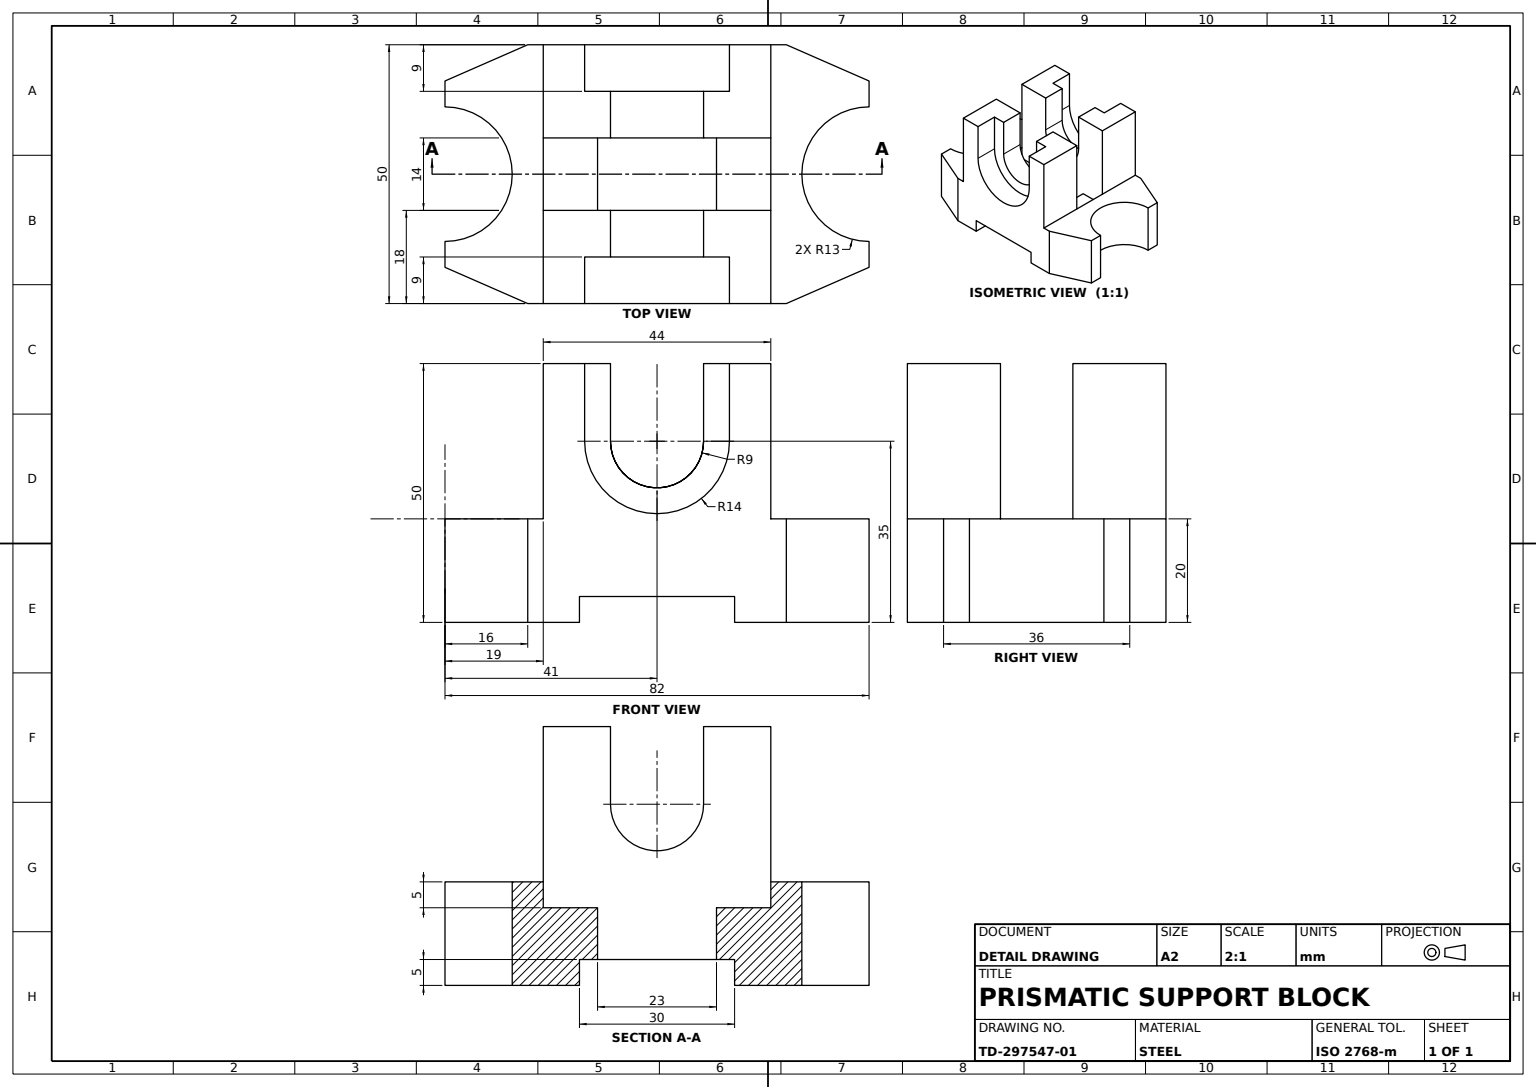
ISO-10303-21;
HEADER;
FILE_DESCRIPTION((''),'2;1');
FILE_NAME('','',(''),(''),'','','');
FILE_SCHEMA(('AUTOMOTIVE_DESIGN'));
ENDSEC;
DATA;
#1=APPLICATION_CONTEXT('');
#2=PRODUCT_CONTEXT('',#1,'mechanical');
#3=PRODUCT('','','',(#2));
#4=PRODUCT_DEFINITION_FORMATION('','',#3);
#5=PRODUCT_DEFINITION_CONTEXT('',#1,'design');
#6=PRODUCT_DEFINITION('','',#4,#5);
#7=PRODUCT_DEFINITION_SHAPE('','',#6);
#8=(LENGTH_UNIT()NAMED_UNIT(*)SI_UNIT(.MILLI.,.METRE.));
#9=(NAMED_UNIT(*)PLANE_ANGLE_UNIT()SI_UNIT($,.RADIAN.));
#10=(NAMED_UNIT(*)SI_UNIT($,.STERADIAN.)SOLID_ANGLE_UNIT());
#11=UNCERTAINTY_MEASURE_WITH_UNIT(LENGTH_MEASURE(1.E-05),#8,'distance_accuracy_value','');
#12=(GEOMETRIC_REPRESENTATION_CONTEXT(3)GLOBAL_UNCERTAINTY_ASSIGNED_CONTEXT((#11))GLOBAL_UNIT_ASSIGNED_CONTEXT((#8,#9,#10))REPRESENTATION_CONTEXT('',''));
#13=CARTESIAN_POINT('',(22.,20.,7.));
#14=VERTEX_POINT('',#13);
#15=CARTESIAN_POINT('',(22.,20.,25.));
#16=VERTEX_POINT('',#15);
#17=DIRECTION('',(0.,0.,1.));
#18=VECTOR('',#17,1000.);
#19=LINE('',#13,#18);
#20=EDGE_CURVE('',#14,#16,#19,.T.);
#21=ORIENTED_EDGE('',*,*,#20,.F.);
#22=CARTESIAN_POINT('',(22.,50.,7.));
#23=VERTEX_POINT('',#22);
#24=DIRECTION('',(0.,1.,0.));
#25=VECTOR('',#24,1000.);
#26=LINE('',#22,#25);
#27=EDGE_CURVE('',#14,#23,#26,.T.);
#28=ORIENTED_EDGE('',*,*,#27,.T.);
#29=CARTESIAN_POINT('',(22.,50.,25.));
#30=VERTEX_POINT('',#29);
#31=LINE('',#22,#18);
#32=EDGE_CURVE('',#23,#30,#31,.T.);
#33=ORIENTED_EDGE('',*,*,#32,.T.);
#34=LINE('',#29,#25);
#35=EDGE_CURVE('',#16,#30,#34,.T.);
#36=ORIENTED_EDGE('',*,*,#35,.F.);
#37=EDGE_LOOP('',(#21,#28,#33,#36));
#38=FACE_OUTER_BOUND('',#37,.T.);
#39=DIRECTION('',(1.,0.,0.));
#40=AXIS2_PLACEMENT_3D('',#22,#39,#24);
#41=PLANE('',#40);
#42=ADVANCED_FACE('',(#38),#41,.T.);
#43=CARTESIAN_POINT('',(14.,35.,-16.));
#44=VERTEX_POINT('',#43);
#45=CARTESIAN_POINT('',(14.,50.,-16.));
#46=VERTEX_POINT('',#45);
#47=LINE('',#45,#25);
#48=EDGE_CURVE('',#44,#46,#47,.T.);
#49=ORIENTED_EDGE('',*,*,#48,.T.);
#50=CARTESIAN_POINT('',(14.,50.,-25.));
#51=VERTEX_POINT('',#50);
#52=DIRECTION('',(0.,0.,-1.));
#53=VECTOR('',#52,1000.);
#54=LINE('',#45,#53);
#55=EDGE_CURVE('',#46,#51,#54,.T.);
#56=ORIENTED_EDGE('',*,*,#55,.T.);
#57=CARTESIAN_POINT('',(14.,35.,-25.));
#58=VERTEX_POINT('',#57);
#59=LINE('',#50,#25);
#60=EDGE_CURVE('',#58,#51,#59,.T.);
#61=ORIENTED_EDGE('',*,*,#60,.F.);
#62=LINE('',#43,#53);
#63=EDGE_CURVE('',#44,#58,#62,.T.);
#64=ORIENTED_EDGE('',*,*,#63,.F.);
#65=EDGE_LOOP('',(#49,#56,#61,#64));
#66=FACE_OUTER_BOUND('',#65,.T.);
#67=DIRECTION('',(-1.,0.,0.));
#68=DIRECTION('',(0.,-1.,0.));
#69=AXIS2_PLACEMENT_3D('',#45,#67,#68);
#70=PLANE('',#69);
#71=ADVANCED_FACE('',(#66),#70,.T.);
#72=CARTESIAN_POINT('',(15.,0.,25.));
#73=VERTEX_POINT('',#72);
#74=CARTESIAN_POINT('',(15.,5.,25.));
#75=VERTEX_POINT('',#74);
#76=CARTESIAN_POINT('',(15.,-5.,25.));
#77=LINE('',#76,#25);
#78=EDGE_CURVE('',#73,#75,#77,.T.);
#79=ORIENTED_EDGE('',*,*,#78,.T.);
#80=CARTESIAN_POINT('',(15.,5.,-25.));
#81=VERTEX_POINT('',#80);
#82=LINE('',#80,#18);
#83=EDGE_CURVE('',#81,#75,#82,.T.);
#84=ORIENTED_EDGE('',*,*,#83,.F.);
#85=CARTESIAN_POINT('',(15.,0.,-25.));
#86=VERTEX_POINT('',#85);
#87=CARTESIAN_POINT('',(15.,-5.,-25.));
#88=LINE('',#87,#25);
#89=EDGE_CURVE('',#86,#81,#88,.T.);
#90=ORIENTED_EDGE('',*,*,#89,.F.);
#91=CARTESIAN_POINT('',(15.,0.,0.));
#92=LINE('',#91,#18);
#93=EDGE_CURVE('',#86,#73,#92,.T.);
#94=ORIENTED_EDGE('',*,*,#93,.T.);
#95=EDGE_LOOP('',(#79,#84,#90,#94));
#96=FACE_OUTER_BOUND('',#95,.T.);
#97=AXIS2_PLACEMENT_3D('',#87,#39,#24);
#98=PLANE('',#97);
#99=ADVANCED_FACE('',(#96),#98,.F.);
#100=CARTESIAN_POINT('',(-22.,50.,-25.));
#101=VERTEX_POINT('',#100);
#102=CARTESIAN_POINT('',(-22.,20.,-25.));
#103=VERTEX_POINT('',#102);
#104=VECTOR('',#68,1000.);
#105=LINE('',#102,#104);
#106=EDGE_CURVE('',#101,#103,#105,.T.);
#107=ORIENTED_EDGE('',*,*,#106,.T.);
#108=CARTESIAN_POINT('',(-22.,20.,-7.));
#109=VERTEX_POINT('',#108);
#110=LINE('',#108,#53);
#111=EDGE_CURVE('',#109,#103,#110,.T.);
#112=ORIENTED_EDGE('',*,*,#111,.F.);
#113=CARTESIAN_POINT('',(-22.,50.,-7.));
#114=VERTEX_POINT('',#113);
#115=LINE('',#108,#104);
#116=EDGE_CURVE('',#114,#109,#115,.T.);
#117=ORIENTED_EDGE('',*,*,#116,.F.);
#118=LINE('',#113,#53);
#119=EDGE_CURVE('',#114,#101,#118,.T.);
#120=ORIENTED_EDGE('',*,*,#119,.T.);
#121=EDGE_LOOP('',(#107,#112,#117,#120));
#122=FACE_OUTER_BOUND('',#121,.T.);
#123=AXIS2_PLACEMENT_3D('',#108,#39,#52);
#124=PLANE('',#123);
#125=ADVANCED_FACE('',(#122),#124,.F.);
#126=CARTESIAN_POINT('',(-22.,15.,7.));
#127=VERTEX_POINT('',#126);
#128=CARTESIAN_POINT('',(-22.,20.,7.));
#129=VERTEX_POINT('',#128);
#130=LINE('',#126,#25);
#131=EDGE_CURVE('',#127,#129,#130,.T.);
#132=ORIENTED_EDGE('',*,*,#131,.F.);
#133=CARTESIAN_POINT('',(-22.,15.,-7.));
#134=VERTEX_POINT('',#133);
#135=LINE('',#133,#18);
#136=EDGE_CURVE('',#134,#127,#135,.T.);
#137=ORIENTED_EDGE('',*,*,#136,.F.);
#138=LINE('',#133,#25);
#139=EDGE_CURVE('',#134,#109,#138,.T.);
#140=ORIENTED_EDGE('',*,*,#139,.T.);
#141=LINE('',#108,#18);
#142=EDGE_CURVE('',#109,#129,#141,.T.);
#143=ORIENTED_EDGE('',*,*,#142,.T.);
#144=EDGE_LOOP('',(#132,#137,#140,#143));
#145=FACE_OUTER_BOUND('',#144,.T.);
#146=AXIS2_PLACEMENT_3D('',#133,#67,#17);
#147=PLANE('',#146);
#148=ADVANCED_FACE('',(#145),#147,.F.);
#149=CARTESIAN_POINT('',(-25.,0.,25.));
#150=VERTEX_POINT('',#149);
#151=CARTESIAN_POINT('',(-15.,0.,25.));
#152=VERTEX_POINT('',#151);
#153=CARTESIAN_POINT('',(25.,0.,25.));
#154=VECTOR('',#39,1000.);
#155=LINE('',#153,#154);
#156=EDGE_CURVE('',#150,#152,#155,.T.);
#157=ORIENTED_EDGE('',*,*,#156,.F.);
#158=CARTESIAN_POINT('',(-41.,0.,18.));
#159=VERTEX_POINT('',#158);
#160=DIRECTION('',(0.916157335,0.,0.400818834));
#161=VECTOR('',#160,1000.);
#162=LINE('',#158,#161);
#163=EDGE_CURVE('',#159,#150,#162,.T.);
#164=ORIENTED_EDGE('',*,*,#163,.F.);
#165=CARTESIAN_POINT('',(-41.,0.,13.));
#166=VERTEX_POINT('',#165);
#167=LINE('',#165,#18);
#168=EDGE_CURVE('',#166,#159,#167,.T.);
#169=ORIENTED_EDGE('',*,*,#168,.F.);
#170=CARTESIAN_POINT('',(-41.,0.,-13.));
#171=VERTEX_POINT('',#170);
#172=CARTESIAN_POINT('',(-41.,0.,0.));
#173=AXIS2_PLACEMENT_3D('',#172,#68,#52);
#174=CIRCLE('',#173,13.);
#175=EDGE_CURVE('',#171,#166,#174,.T.);
#176=ORIENTED_EDGE('',*,*,#175,.F.);
#177=CARTESIAN_POINT('',(-41.,0.,-18.));
#178=VERTEX_POINT('',#177);
#179=LINE('',#177,#18);
#180=EDGE_CURVE('',#178,#171,#179,.T.);
#181=ORIENTED_EDGE('',*,*,#180,.F.);
#182=CARTESIAN_POINT('',(-25.,0.,-25.));
#183=VERTEX_POINT('',#182);
#184=DIRECTION('',(-0.916157335,0.,0.400818834));
#185=VECTOR('',#184,1000.);
#186=LINE('',#182,#185);
#187=EDGE_CURVE('',#183,#178,#186,.T.);
#188=ORIENTED_EDGE('',*,*,#187,.F.);
#189=CARTESIAN_POINT('',(-15.,0.,-25.));
#190=VERTEX_POINT('',#189);
#191=VECTOR('',#67,1000.);
#192=LINE('',#182,#191);
#193=EDGE_CURVE('',#190,#183,#192,.T.);
#194=ORIENTED_EDGE('',*,*,#193,.F.);
#195=CARTESIAN_POINT('',(-15.,0.,0.));
#196=LINE('',#195,#53);
#197=EDGE_CURVE('',#152,#190,#196,.T.);
#198=ORIENTED_EDGE('',*,*,#197,.F.);
#199=EDGE_LOOP('',(#157,#164,#169,#176,#181,#188,#194,#198));
#200=FACE_OUTER_BOUND('',#199,.T.);
#201=PLANE('',#173);
#202=ADVANCED_FACE('',(#200),#201,.T.);
#203=VERTEX_POINT('',#153);
#204=EDGE_CURVE('',#73,#203,#155,.T.);
#205=ORIENTED_EDGE('',*,*,#204,.T.);
#206=CARTESIAN_POINT('',(25.,20.,25.));
#207=VERTEX_POINT('',#206);
#208=LINE('',#206,#104);
#209=EDGE_CURVE('',#207,#203,#208,.T.);
#210=ORIENTED_EDGE('',*,*,#209,.F.);
#211=LINE('',#206,#154);
#212=EDGE_CURVE('',#16,#207,#211,.T.);
#213=ORIENTED_EDGE('',*,*,#212,.F.);
#214=ORIENTED_EDGE('',*,*,#35,.T.);
#215=CARTESIAN_POINT('',(14.,50.,25.));
#216=VERTEX_POINT('',#215);
#217=CARTESIAN_POINT('',(9.,50.,25.));
#218=LINE('',#217,#191);
#219=EDGE_CURVE('',#30,#216,#218,.T.);
#220=ORIENTED_EDGE('',*,*,#219,.T.);
#221=CARTESIAN_POINT('',(14.,35.,25.));
#222=VERTEX_POINT('',#221);
#223=LINE('',#215,#25);
#224=EDGE_CURVE('',#222,#216,#223,.T.);
#225=ORIENTED_EDGE('',*,*,#224,.F.);
#226=CARTESIAN_POINT('',(-14.,35.,25.));
#227=VERTEX_POINT('',#226);
#228=CARTESIAN_POINT('',(0.,35.,25.));
#229=AXIS2_PLACEMENT_3D('',#228,#17,#39);
#230=CIRCLE('',#229,14.);
#231=EDGE_CURVE('',#227,#222,#230,.T.);
#232=ORIENTED_EDGE('',*,*,#231,.F.);
#233=CARTESIAN_POINT('',(-14.,50.,25.));
#234=VERTEX_POINT('',#233);
#235=LINE('',#226,#104);
#236=EDGE_CURVE('',#234,#227,#235,.T.);
#237=ORIENTED_EDGE('',*,*,#236,.F.);
#238=CARTESIAN_POINT('',(-22.,50.,25.));
#239=VERTEX_POINT('',#238);
#240=LINE('',#238,#191);
#241=EDGE_CURVE('',#234,#239,#240,.T.);
#242=ORIENTED_EDGE('',*,*,#241,.T.);
#243=CARTESIAN_POINT('',(-22.,20.,25.));
#244=VERTEX_POINT('',#243);
#245=LINE('',#243,#104);
#246=EDGE_CURVE('',#239,#244,#245,.T.);
#247=ORIENTED_EDGE('',*,*,#246,.T.);
#248=CARTESIAN_POINT('',(-25.,20.,25.));
#249=VERTEX_POINT('',#248);
#250=EDGE_CURVE('',#249,#244,#211,.T.);
#251=ORIENTED_EDGE('',*,*,#250,.F.);
#252=LINE('',#248,#104);
#253=EDGE_CURVE('',#249,#150,#252,.T.);
#254=ORIENTED_EDGE('',*,*,#253,.T.);
#255=ORIENTED_EDGE('',*,*,#156,.T.);
#256=CARTESIAN_POINT('',(-15.,5.,25.));
#257=VERTEX_POINT('',#256);
#258=CARTESIAN_POINT('',(-15.,-5.,25.));
#259=LINE('',#258,#104);
#260=EDGE_CURVE('',#257,#152,#259,.T.);
#261=ORIENTED_EDGE('',*,*,#260,.F.);
#262=LINE('',#256,#191);
#263=EDGE_CURVE('',#75,#257,#262,.T.);
#264=ORIENTED_EDGE('',*,*,#263,.F.);
#265=ORIENTED_EDGE('',*,*,#78,.F.);
#266=EDGE_LOOP('',(#205,#210,#213,#214,#220,#225,#232,#237,#242,#247,#251,#254,#255,#261,#264,#265));
#267=FACE_OUTER_BOUND('',#266,.T.);
#268=AXIS2_PLACEMENT_3D('',#206,#52,#67);
#269=PLANE('',#268);
#270=ADVANCED_FACE('',(#267),#269,.F.);
#271=CARTESIAN_POINT('',(-11.5,5.,7.));
#272=VERTEX_POINT('',#271);
#273=CARTESIAN_POINT('',(-11.5,15.,7.));
#274=VERTEX_POINT('',#273);
#275=CARTESIAN_POINT('',(-11.5,0.,7.));
#276=LINE('',#275,#25);
#277=EDGE_CURVE('',#272,#274,#276,.T.);
#278=ORIENTED_EDGE('',*,*,#277,.F.);
#279=CARTESIAN_POINT('',(-11.5,5.,-7.));
#280=VERTEX_POINT('',#279);
#281=CARTESIAN_POINT('',(-11.5,5.,-25.));
#282=LINE('',#281,#18);
#283=EDGE_CURVE('',#280,#272,#282,.T.);
#284=ORIENTED_EDGE('',*,*,#283,.F.);
#285=CARTESIAN_POINT('',(-11.5,15.,-7.));
#286=VERTEX_POINT('',#285);
#287=CARTESIAN_POINT('',(-11.5,0.,-7.));
#288=LINE('',#287,#25);
#289=EDGE_CURVE('',#280,#286,#288,.T.);
#290=ORIENTED_EDGE('',*,*,#289,.T.);
#291=LINE('',#273,#53);
#292=EDGE_CURVE('',#274,#286,#291,.T.);
#293=ORIENTED_EDGE('',*,*,#292,.F.);
#294=EDGE_LOOP('',(#278,#284,#290,#293));
#295=FACE_OUTER_BOUND('',#294,.T.);
#296=AXIS2_PLACEMENT_3D('',#275,#67,#17);
#297=PLANE('',#296);
#298=ADVANCED_FACE('',(#295),#297,.F.);
#299=CARTESIAN_POINT('',(9.,35.,-16.));
#300=VERTEX_POINT('',#299);
#301=CARTESIAN_POINT('',(9.,50.,-16.));
#302=VERTEX_POINT('',#301);
#303=LINE('',#299,#25);
#304=EDGE_CURVE('',#300,#302,#303,.T.);
#305=ORIENTED_EDGE('',*,*,#304,.F.);
#306=CARTESIAN_POINT('',(9.,35.,-7.));
#307=VERTEX_POINT('',#306);
#308=LINE('',#306,#53);
#309=EDGE_CURVE('',#307,#300,#308,.T.);
#310=ORIENTED_EDGE('',*,*,#309,.F.);
#311=CARTESIAN_POINT('',(9.,50.,-7.));
#312=VERTEX_POINT('',#311);
#313=LINE('',#306,#104);
#314=EDGE_CURVE('',#312,#307,#313,.T.);
#315=ORIENTED_EDGE('',*,*,#314,.F.);
#316=LINE('',#311,#53);
#317=EDGE_CURVE('',#312,#302,#316,.T.);
#318=ORIENTED_EDGE('',*,*,#317,.T.);
#319=EDGE_LOOP('',(#305,#310,#315,#318));
#320=FACE_OUTER_BOUND('',#319,.T.);
#321=AXIS2_PLACEMENT_3D('',#306,#39,#24);
#322=PLANE('',#321);
#323=ADVANCED_FACE('',(#320),#322,.F.);
#324=CARTESIAN_POINT('',(22.,15.,-7.));
#325=VERTEX_POINT('',#324);
#326=CARTESIAN_POINT('',(22.,20.,-7.));
#327=VERTEX_POINT('',#326);
#328=LINE('',#324,#25);
#329=EDGE_CURVE('',#325,#327,#328,.T.);
#330=ORIENTED_EDGE('',*,*,#329,.F.);
#331=CARTESIAN_POINT('',(22.,15.,7.));
#332=VERTEX_POINT('',#331);
#333=LINE('',#324,#53);
#334=EDGE_CURVE('',#332,#325,#333,.T.);
#335=ORIENTED_EDGE('',*,*,#334,.F.);
#336=LINE('',#331,#25);
#337=EDGE_CURVE('',#332,#14,#336,.T.);
#338=ORIENTED_EDGE('',*,*,#337,.T.);
#339=LINE('',#326,#53);
#340=EDGE_CURVE('',#14,#327,#339,.T.);
#341=ORIENTED_EDGE('',*,*,#340,.T.);
#342=EDGE_LOOP('',(#330,#335,#338,#341));
#343=FACE_OUTER_BOUND('',#342,.T.);
#344=AXIS2_PLACEMENT_3D('',#324,#39,#52);
#345=PLANE('',#344);
#346=ADVANCED_FACE('',(#343),#345,.F.);
#347=CARTESIAN_POINT('',(9.,50.,7.));
#348=VERTEX_POINT('',#347);
#349=CARTESIAN_POINT('',(9.,50.,16.));
#350=VERTEX_POINT('',#349);
#351=LINE('',#347,#18);
#352=EDGE_CURVE('',#348,#350,#351,.T.);
#353=ORIENTED_EDGE('',*,*,#352,.F.);
#354=CARTESIAN_POINT('',(9.,35.,7.));
#355=VERTEX_POINT('',#354);
#356=LINE('',#354,#104);
#357=EDGE_CURVE('',#348,#355,#356,.T.);
#358=ORIENTED_EDGE('',*,*,#357,.T.);
#359=CARTESIAN_POINT('',(9.,35.,16.));
#360=VERTEX_POINT('',#359);
#361=LINE('',#354,#18);
#362=EDGE_CURVE('',#355,#360,#361,.T.);
#363=ORIENTED_EDGE('',*,*,#362,.T.);
#364=LINE('',#359,#25);
#365=EDGE_CURVE('',#360,#350,#364,.T.);
#366=ORIENTED_EDGE('',*,*,#365,.T.);
#367=EDGE_LOOP('',(#353,#358,#363,#366));
#368=FACE_OUTER_BOUND('',#367,.T.);
#369=AXIS2_PLACEMENT_3D('',#354,#67,#68);
#370=PLANE('',#369);
#371=ADVANCED_FACE('',(#368),#370,.T.);
#372=CARTESIAN_POINT('',(-9.,50.,7.));
#373=VERTEX_POINT('',#372);
#374=CARTESIAN_POINT('',(-9.,50.,16.));
#375=VERTEX_POINT('',#374);
#376=LINE('',#372,#18);
#377=EDGE_CURVE('',#373,#375,#376,.T.);
#378=ORIENTED_EDGE('',*,*,#377,.T.);
#379=CARTESIAN_POINT('',(-9.,35.,16.));
#380=VERTEX_POINT('',#379);
#381=LINE('',#374,#104);
#382=EDGE_CURVE('',#375,#380,#381,.T.);
#383=ORIENTED_EDGE('',*,*,#382,.T.);
#384=CARTESIAN_POINT('',(-9.,35.,7.));
#385=VERTEX_POINT('',#384);
#386=LINE('',#384,#18);
#387=EDGE_CURVE('',#385,#380,#386,.T.);
#388=ORIENTED_EDGE('',*,*,#387,.F.);
#389=LINE('',#372,#25);
#390=EDGE_CURVE('',#385,#373,#389,.T.);
#391=ORIENTED_EDGE('',*,*,#390,.T.);
#392=EDGE_LOOP('',(#378,#383,#388,#391));
#393=FACE_OUTER_BOUND('',#392,.T.);
#394=AXIS2_PLACEMENT_3D('',#372,#39,#24);
#395=PLANE('',#394);
#396=ADVANCED_FACE('',(#393),#395,.T.);
#397=CARTESIAN_POINT('',(14.,50.,16.));
#398=VERTEX_POINT('',#397);
#399=CARTESIAN_POINT('',(-14.,50.,16.));
#400=LINE('',#399,#191);
#401=EDGE_CURVE('',#398,#350,#400,.T.);
#402=ORIENTED_EDGE('',*,*,#401,.F.);
#403=LINE('',#397,#18);
#404=EDGE_CURVE('',#398,#216,#403,.T.);
#405=ORIENTED_EDGE('',*,*,#404,.T.);
#406=ORIENTED_EDGE('',*,*,#219,.F.);
#407=ORIENTED_EDGE('',*,*,#32,.F.);
#408=LINE('',#347,#191);
#409=EDGE_CURVE('',#23,#348,#408,.T.);
#410=ORIENTED_EDGE('',*,*,#409,.T.);
#411=ORIENTED_EDGE('',*,*,#352,.T.);
#412=EDGE_LOOP('',(#402,#405,#406,#407,#410,#411));
#413=FACE_OUTER_BOUND('',#412,.T.);
#414=AXIS2_PLACEMENT_3D('',#347,#24,#17);
#415=PLANE('',#414);
#416=ADVANCED_FACE('',(#413),#415,.T.);
#417=CARTESIAN_POINT('',(41.,0.,13.));
#418=VERTEX_POINT('',#417);
#419=CARTESIAN_POINT('',(41.,0.,-13.));
#420=VERTEX_POINT('',#419);
#421=CARTESIAN_POINT('',(41.,0.,0.));
#422=AXIS2_PLACEMENT_3D('',#421,#68,#17);
#423=CIRCLE('',#422,13.);
#424=EDGE_CURVE('',#418,#420,#423,.T.);
#425=ORIENTED_EDGE('',*,*,#424,.T.);
#426=CARTESIAN_POINT('',(41.,20.,-13.));
#427=VERTEX_POINT('',#426);
#428=LINE('',#426,#104);
#429=EDGE_CURVE('',#427,#420,#428,.T.);
#430=ORIENTED_EDGE('',*,*,#429,.F.);
#431=CARTESIAN_POINT('',(41.,20.,13.));
#432=VERTEX_POINT('',#431);
#433=CARTESIAN_POINT('',(41.,20.,0.));
#434=AXIS2_PLACEMENT_3D('',#433,#68,#17);
#435=CIRCLE('',#434,13.);
#436=EDGE_CURVE('',#432,#427,#435,.T.);
#437=ORIENTED_EDGE('',*,*,#436,.F.);
#438=LINE('',#431,#104);
#439=EDGE_CURVE('',#432,#418,#438,.T.);
#440=ORIENTED_EDGE('',*,*,#439,.T.);
#441=EDGE_LOOP('',(#425,#430,#437,#440));
#442=FACE_OUTER_BOUND('',#441,.T.);
#443=AXIS2_PLACEMENT_3D('',#433,#68,#52);
#444=CYLINDRICAL_SURFACE('',#443,13.);
#445=ADVANCED_FACE('',(#442),#444,.F.);
#446=CARTESIAN_POINT('',(22.,20.,-25.));
#447=VERTEX_POINT('',#446);
#448=CARTESIAN_POINT('',(22.,50.,-25.));
#449=VERTEX_POINT('',#448);
#450=LINE('',#448,#25);
#451=EDGE_CURVE('',#447,#449,#450,.T.);
#452=ORIENTED_EDGE('',*,*,#451,.T.);
#453=CARTESIAN_POINT('',(22.,50.,-7.));
#454=VERTEX_POINT('',#453);
#455=LINE('',#453,#53);
#456=EDGE_CURVE('',#454,#449,#455,.T.);
#457=ORIENTED_EDGE('',*,*,#456,.F.);
#458=LINE('',#453,#25);
#459=EDGE_CURVE('',#327,#454,#458,.T.);
#460=ORIENTED_EDGE('',*,*,#459,.F.);
#461=EDGE_CURVE('',#327,#447,#339,.T.);
#462=ORIENTED_EDGE('',*,*,#461,.T.);
#463=EDGE_LOOP('',(#452,#457,#460,#462));
#464=FACE_OUTER_BOUND('',#463,.T.);
#465=AXIS2_PLACEMENT_3D('',#453,#67,#68);
#466=PLANE('',#465);
#467=ADVANCED_FACE('',(#464),#466,.F.);
#468=CARTESIAN_POINT('',(11.5,15.,-7.));
#469=VERTEX_POINT('',#468);
#470=CARTESIAN_POINT('',(11.5,15.,7.));
#471=VERTEX_POINT('',#470);
#472=LINE('',#470,#18);
#473=EDGE_CURVE('',#469,#471,#472,.T.);
#474=ORIENTED_EDGE('',*,*,#473,.F.);
#475=CARTESIAN_POINT('',(11.5,5.,-7.));
#476=VERTEX_POINT('',#475);
#477=CARTESIAN_POINT('',(11.5,0.,-7.));
#478=LINE('',#477,#25);
#479=EDGE_CURVE('',#476,#469,#478,.T.);
#480=ORIENTED_EDGE('',*,*,#479,.F.);
#481=CARTESIAN_POINT('',(11.5,5.,7.));
#482=VERTEX_POINT('',#481);
#483=CARTESIAN_POINT('',(11.5,5.,-25.));
#484=LINE('',#483,#53);
#485=EDGE_CURVE('',#482,#476,#484,.T.);
#486=ORIENTED_EDGE('',*,*,#485,.F.);
#487=CARTESIAN_POINT('',(11.5,0.,7.));
#488=LINE('',#487,#25);
#489=EDGE_CURVE('',#482,#471,#488,.T.);
#490=ORIENTED_EDGE('',*,*,#489,.T.);
#491=EDGE_LOOP('',(#474,#480,#486,#490));
#492=FACE_OUTER_BOUND('',#491,.T.);
#493=AXIS2_PLACEMENT_3D('',#487,#39,#52);
#494=PLANE('',#493);
#495=ADVANCED_FACE('',(#492),#494,.F.);
#496=ORIENTED_EDGE('',*,*,#163,.T.);
#497=ORIENTED_EDGE('',*,*,#253,.F.);
#498=CARTESIAN_POINT('',(-41.,20.,18.));
#499=VERTEX_POINT('',#498);
#500=LINE('',#498,#161);
#501=EDGE_CURVE('',#499,#249,#500,.T.);
#502=ORIENTED_EDGE('',*,*,#501,.F.);
#503=LINE('',#498,#104);
#504=EDGE_CURVE('',#499,#159,#503,.T.);
#505=ORIENTED_EDGE('',*,*,#504,.T.);
#506=EDGE_LOOP('',(#496,#497,#502,#505));
#507=FACE_OUTER_BOUND('',#506,.T.);
#508=DIRECTION('',(0.400818834,0.,-0.916157335));
#509=DIRECTION('',(-0.916157335,0.,-0.400818834));
#510=AXIS2_PLACEMENT_3D('',#498,#508,#509);
#511=PLANE('',#510);
#512=ADVANCED_FACE('',(#507),#511,.F.);
#513=CARTESIAN_POINT('',(-14.,35.,16.));
#514=VERTEX_POINT('',#513);
#515=LINE('',#513,#18);
#516=EDGE_CURVE('',#514,#227,#515,.T.);
#517=ORIENTED_EDGE('',*,*,#516,.T.);
#518=ORIENTED_EDGE('',*,*,#231,.T.);
#519=CARTESIAN_POINT('',(14.,35.,16.));
#520=VERTEX_POINT('',#519);
#521=LINE('',#519,#18);
#522=EDGE_CURVE('',#520,#222,#521,.T.);
#523=ORIENTED_EDGE('',*,*,#522,.F.);
#524=CARTESIAN_POINT('',(0.,35.,16.));
#525=AXIS2_PLACEMENT_3D('',#524,#17,#39);
#526=CIRCLE('',#525,14.);
#527=EDGE_CURVE('',#514,#520,#526,.T.);
#528=ORIENTED_EDGE('',*,*,#527,.F.);
#529=EDGE_LOOP('',(#517,#518,#523,#528));
#530=FACE_OUTER_BOUND('',#529,.T.);
#531=CYLINDRICAL_SURFACE('',#525,14.);
#532=ADVANCED_FACE('',(#530),#531,.F.);
#533=CARTESIAN_POINT('',(-15.,5.,-25.));
#534=VERTEX_POINT('',#533);
#535=LINE('',#533,#18);
#536=EDGE_CURVE('',#534,#257,#535,.T.);
#537=ORIENTED_EDGE('',*,*,#536,.F.);
#538=LINE('',#533,#191);
#539=EDGE_CURVE('',#81,#534,#538,.T.);
#540=ORIENTED_EDGE('',*,*,#539,.F.);
#541=ORIENTED_EDGE('',*,*,#83,.T.);
#542=ORIENTED_EDGE('',*,*,#263,.T.);
#543=EDGE_LOOP('',(#537,#540,#541,#542));
#544=FACE_OUTER_BOUND('',#543,.T.);
#545=CARTESIAN_POINT('',(-15.,5.,7.));
#546=LINE('',#545,#154);
#547=EDGE_CURVE('',#272,#482,#546,.T.);
#548=ORIENTED_EDGE('',*,*,#547,.T.);
#549=ORIENTED_EDGE('',*,*,#485,.T.);
#550=CARTESIAN_POINT('',(-15.,5.,-7.));
#551=LINE('',#550,#191);
#552=EDGE_CURVE('',#476,#280,#551,.T.);
#553=ORIENTED_EDGE('',*,*,#552,.T.);
#554=ORIENTED_EDGE('',*,*,#283,.T.);
#555=EDGE_LOOP('',(#548,#549,#553,#554));
#556=FACE_BOUND('',#555,.T.);
#557=AXIS2_PLACEMENT_3D('',#533,#24,#17);
#558=PLANE('',#557);
#559=ADVANCED_FACE('',(#544,#556),#558,.F.);
#560=ORIENTED_EDGE('',*,*,#197,.T.);
#561=CARTESIAN_POINT('',(-15.,-5.,-25.));
#562=LINE('',#561,#104);
#563=EDGE_CURVE('',#534,#190,#562,.T.);
#564=ORIENTED_EDGE('',*,*,#563,.F.);
#565=ORIENTED_EDGE('',*,*,#536,.T.);
#566=ORIENTED_EDGE('',*,*,#260,.T.);
#567=EDGE_LOOP('',(#560,#564,#565,#566));
#568=FACE_OUTER_BOUND('',#567,.T.);
#569=AXIS2_PLACEMENT_3D('',#561,#67,#68);
#570=PLANE('',#569);
#571=ADVANCED_FACE('',(#568),#570,.F.);
#572=CARTESIAN_POINT('',(-41.,20.,13.));
#573=VERTEX_POINT('',#572);
#574=LINE('',#572,#104);
#575=EDGE_CURVE('',#573,#166,#574,.T.);
#576=ORIENTED_EDGE('',*,*,#575,.T.);
#577=ORIENTED_EDGE('',*,*,#168,.T.);
#578=ORIENTED_EDGE('',*,*,#504,.F.);
#579=LINE('',#572,#18);
#580=EDGE_CURVE('',#573,#499,#579,.T.);
#581=ORIENTED_EDGE('',*,*,#580,.F.);
#582=EDGE_LOOP('',(#576,#577,#578,#581));
#583=FACE_OUTER_BOUND('',#582,.T.);
#584=AXIS2_PLACEMENT_3D('',#572,#39,#52);
#585=PLANE('',#584);
#586=ADVANCED_FACE('',(#583),#585,.F.);
#587=ORIENTED_EDGE('',*,*,#516,.F.);
#588=VERTEX_POINT('',#399);
#589=LINE('',#513,#104);
#590=EDGE_CURVE('',#588,#514,#589,.T.);
#591=ORIENTED_EDGE('',*,*,#590,.F.);
#592=LINE('',#399,#18);
#593=EDGE_CURVE('',#588,#234,#592,.T.);
#594=ORIENTED_EDGE('',*,*,#593,.T.);
#595=ORIENTED_EDGE('',*,*,#236,.T.);
#596=EDGE_LOOP('',(#587,#591,#594,#595));
#597=FACE_OUTER_BOUND('',#596,.T.);
#598=AXIS2_PLACEMENT_3D('',#513,#67,#68);
#599=PLANE('',#598);
#600=ADVANCED_FACE('',(#597),#599,.F.);
#601=CARTESIAN_POINT('',(41.,20.,18.));
#602=VERTEX_POINT('',#601);
#603=LINE('',#431,#53);
#604=EDGE_CURVE('',#602,#432,#603,.T.);
#605=ORIENTED_EDGE('',*,*,#604,.F.);
#606=CARTESIAN_POINT('',(41.,0.,18.));
#607=VERTEX_POINT('',#606);
#608=LINE('',#601,#104);
#609=EDGE_CURVE('',#602,#607,#608,.T.);
#610=ORIENTED_EDGE('',*,*,#609,.T.);
#611=LINE('',#417,#53);
#612=EDGE_CURVE('',#607,#418,#611,.T.);
#613=ORIENTED_EDGE('',*,*,#612,.T.);
#614=ORIENTED_EDGE('',*,*,#439,.F.);
#615=EDGE_LOOP('',(#605,#610,#613,#614));
#616=FACE_OUTER_BOUND('',#615,.T.);
#617=AXIS2_PLACEMENT_3D('',#431,#67,#17);
#618=PLANE('',#617);
#619=ADVANCED_FACE('',(#616),#618,.F.);
#620=CARTESIAN_POINT('',(-22.,50.,7.));
#621=VERTEX_POINT('',#620);
#622=LINE('',#128,#104);
#623=EDGE_CURVE('',#621,#129,#622,.T.);
#624=ORIENTED_EDGE('',*,*,#623,.T.);
#625=LINE('',#128,#18);
#626=EDGE_CURVE('',#129,#244,#625,.T.);
#627=ORIENTED_EDGE('',*,*,#626,.T.);
#628=ORIENTED_EDGE('',*,*,#246,.F.);
#629=LINE('',#620,#18);
#630=EDGE_CURVE('',#621,#239,#629,.T.);
#631=ORIENTED_EDGE('',*,*,#630,.F.);
#632=EDGE_LOOP('',(#624,#627,#628,#631));
#633=FACE_OUTER_BOUND('',#632,.T.);
#634=AXIS2_PLACEMENT_3D('',#128,#67,#17);
#635=PLANE('',#634);
#636=ADVANCED_FACE('',(#633),#635,.T.);
#637=CARTESIAN_POINT('',(-25.,20.,-25.));
#638=VERTEX_POINT('',#637);
#639=LINE('',#637,#104);
#640=EDGE_CURVE('',#638,#183,#639,.T.);
#641=ORIENTED_EDGE('',*,*,#640,.T.);
#642=ORIENTED_EDGE('',*,*,#187,.T.);
#643=CARTESIAN_POINT('',(-41.,20.,-18.));
#644=VERTEX_POINT('',#643);
#645=LINE('',#643,#104);
#646=EDGE_CURVE('',#644,#178,#645,.T.);
#647=ORIENTED_EDGE('',*,*,#646,.F.);
#648=LINE('',#637,#185);
#649=EDGE_CURVE('',#638,#644,#648,.T.);
#650=ORIENTED_EDGE('',*,*,#649,.F.);
#651=EDGE_LOOP('',(#641,#642,#647,#650));
#652=FACE_OUTER_BOUND('',#651,.T.);
#653=DIRECTION('',(0.400818834,0.,0.916157335));
#654=DIRECTION('',(0.916157335,0.,-0.400818834));
#655=AXIS2_PLACEMENT_3D('',#637,#653,#654);
#656=PLANE('',#655);
#657=ADVANCED_FACE('',(#652),#656,.F.);
#658=CARTESIAN_POINT('',(-41.,20.,-13.));
#659=VERTEX_POINT('',#658);
#660=LINE('',#643,#18);
#661=EDGE_CURVE('',#644,#659,#660,.T.);
#662=ORIENTED_EDGE('',*,*,#661,.F.);
#663=ORIENTED_EDGE('',*,*,#646,.T.);
#664=ORIENTED_EDGE('',*,*,#180,.T.);
#665=LINE('',#658,#104);
#666=EDGE_CURVE('',#659,#171,#665,.T.);
#667=ORIENTED_EDGE('',*,*,#666,.F.);
#668=EDGE_LOOP('',(#662,#663,#664,#667));
#669=FACE_OUTER_BOUND('',#668,.T.);
#670=AXIS2_PLACEMENT_3D('',#643,#39,#52);
#671=PLANE('',#670);
#672=ADVANCED_FACE('',(#669),#671,.F.);
#673=ORIENTED_EDGE('',*,*,#387,.T.);
#674=CIRCLE('',#525,9.);
#675=EDGE_CURVE('',#380,#360,#674,.T.);
#676=ORIENTED_EDGE('',*,*,#675,.T.);
#677=ORIENTED_EDGE('',*,*,#362,.F.);
#678=CARTESIAN_POINT('',(0.,35.,7.));
#679=AXIS2_PLACEMENT_3D('',#678,#52,#39);
#680=CIRCLE('',#679,9.);
#681=EDGE_CURVE('',#355,#385,#680,.T.);
#682=ORIENTED_EDGE('',*,*,#681,.T.);
#683=EDGE_LOOP('',(#673,#676,#677,#682));
#684=FACE_OUTER_BOUND('',#683,.T.);
#685=AXIS2_PLACEMENT_3D('',#678,#17,#39);
#686=CYLINDRICAL_SURFACE('',#685,9.);
#687=ADVANCED_FACE('',(#684),#686,.F.);
#688=CARTESIAN_POINT('',(9.,50.,-25.));
#689=LINE('',#688,#191);
#690=EDGE_CURVE('',#449,#51,#689,.T.);
#691=ORIENTED_EDGE('',*,*,#690,.T.);
#692=ORIENTED_EDGE('',*,*,#55,.F.);
#693=CARTESIAN_POINT('',(-14.,50.,-16.));
#694=LINE('',#693,#191);
#695=EDGE_CURVE('',#46,#302,#694,.T.);
#696=ORIENTED_EDGE('',*,*,#695,.T.);
#697=ORIENTED_EDGE('',*,*,#317,.F.);
#698=LINE('',#311,#191);
#699=EDGE_CURVE('',#454,#312,#698,.T.);
#700=ORIENTED_EDGE('',*,*,#699,.F.);
#701=ORIENTED_EDGE('',*,*,#456,.T.);
#702=EDGE_LOOP('',(#691,#692,#696,#697,#700,#701));
#703=FACE_OUTER_BOUND('',#702,.T.);
#704=AXIS2_PLACEMENT_3D('',#311,#68,#52);
#705=PLANE('',#704);
#706=ADVANCED_FACE('',(#703),#705,.F.);
#707=CARTESIAN_POINT('',(-9.,35.,-7.));
#708=VERTEX_POINT('',#707);
#709=CARTESIAN_POINT('',(0.,35.,-7.));
#710=AXIS2_PLACEMENT_3D('',#709,#52,#39);
#711=CIRCLE('',#710,9.);
#712=EDGE_CURVE('',#307,#708,#711,.T.);
#713=ORIENTED_EDGE('',*,*,#712,.F.);
#714=ORIENTED_EDGE('',*,*,#309,.T.);
#715=CARTESIAN_POINT('',(-9.,35.,-16.));
#716=VERTEX_POINT('',#715);
#717=CARTESIAN_POINT('',(0.,35.,-16.));
#718=AXIS2_PLACEMENT_3D('',#717,#17,#67);
#719=CIRCLE('',#718,9.);
#720=EDGE_CURVE('',#716,#300,#719,.T.);
#721=ORIENTED_EDGE('',*,*,#720,.F.);
#722=LINE('',#707,#53);
#723=EDGE_CURVE('',#708,#716,#722,.T.);
#724=ORIENTED_EDGE('',*,*,#723,.F.);
#725=EDGE_LOOP('',(#713,#714,#721,#724));
#726=FACE_OUTER_BOUND('',#725,.T.);
#727=AXIS2_PLACEMENT_3D('',#709,#52,#67);
#728=CYLINDRICAL_SURFACE('',#727,9.);
#729=ADVANCED_FACE('',(#726),#728,.F.);
#730=VECTOR('',#654,1000.);
#731=LINE('',#601,#730);
#732=EDGE_CURVE('',#207,#602,#731,.T.);
#733=ORIENTED_EDGE('',*,*,#732,.F.);
#734=ORIENTED_EDGE('',*,*,#209,.T.);
#735=LINE('',#606,#730);
#736=EDGE_CURVE('',#203,#607,#735,.T.);
#737=ORIENTED_EDGE('',*,*,#736,.T.);
#738=ORIENTED_EDGE('',*,*,#609,.F.);
#739=EDGE_LOOP('',(#733,#734,#737,#738));
#740=FACE_OUTER_BOUND('',#739,.T.);
#741=DIRECTION('',(-0.400818834,0.,-0.916157335));
#742=AXIS2_PLACEMENT_3D('',#601,#741,#184);
#743=PLANE('',#742);
#744=ADVANCED_FACE('',(#740),#743,.F.);
#745=VERTEX_POINT('',#693);
#746=CARTESIAN_POINT('',(-14.,50.,-25.));
#747=VERTEX_POINT('',#746);
#748=LINE('',#693,#53);
#749=EDGE_CURVE('',#745,#747,#748,.T.);
#750=ORIENTED_EDGE('',*,*,#749,.T.);
#751=LINE('',#100,#191);
#752=EDGE_CURVE('',#747,#101,#751,.T.);
#753=ORIENTED_EDGE('',*,*,#752,.T.);
#754=ORIENTED_EDGE('',*,*,#119,.F.);
#755=CARTESIAN_POINT('',(-9.,50.,-7.));
#756=VERTEX_POINT('',#755);
#757=LINE('',#113,#191);
#758=EDGE_CURVE('',#756,#114,#757,.T.);
#759=ORIENTED_EDGE('',*,*,#758,.F.);
#760=CARTESIAN_POINT('',(-9.,50.,-16.));
#761=VERTEX_POINT('',#760);
#762=LINE('',#755,#53);
#763=EDGE_CURVE('',#756,#761,#762,.T.);
#764=ORIENTED_EDGE('',*,*,#763,.T.);
#765=CARTESIAN_POINT('',(-22.,50.,-16.));
#766=LINE('',#765,#154);
#767=EDGE_CURVE('',#745,#761,#766,.T.);
#768=ORIENTED_EDGE('',*,*,#767,.F.);
#769=EDGE_LOOP('',(#750,#753,#754,#759,#764,#768));
#770=FACE_OUTER_BOUND('',#769,.T.);
#771=AXIS2_PLACEMENT_3D('',#113,#68,#52);
#772=PLANE('',#771);
#773=ADVANCED_FACE('',(#770),#772,.F.);
#774=ORIENTED_EDGE('',*,*,#690,.F.);
#775=ORIENTED_EDGE('',*,*,#451,.F.);
#776=CARTESIAN_POINT('',(25.,20.,-25.));
#777=VERTEX_POINT('',#776);
#778=LINE('',#637,#191);
#779=EDGE_CURVE('',#777,#447,#778,.T.);
#780=ORIENTED_EDGE('',*,*,#779,.F.);
#781=CARTESIAN_POINT('',(25.,0.,-25.));
#782=VERTEX_POINT('',#781);
#783=LINE('',#776,#104);
#784=EDGE_CURVE('',#777,#782,#783,.T.);
#785=ORIENTED_EDGE('',*,*,#784,.T.);
#786=EDGE_CURVE('',#782,#86,#192,.T.);
#787=ORIENTED_EDGE('',*,*,#786,.T.);
#788=ORIENTED_EDGE('',*,*,#89,.T.);
#789=ORIENTED_EDGE('',*,*,#539,.T.);
#790=ORIENTED_EDGE('',*,*,#563,.T.);
#791=ORIENTED_EDGE('',*,*,#193,.T.);
#792=ORIENTED_EDGE('',*,*,#640,.F.);
#793=EDGE_CURVE('',#103,#638,#778,.T.);
#794=ORIENTED_EDGE('',*,*,#793,.F.);
#795=ORIENTED_EDGE('',*,*,#106,.F.);
#796=ORIENTED_EDGE('',*,*,#752,.F.);
#797=CARTESIAN_POINT('',(-14.,35.,-25.));
#798=VERTEX_POINT('',#797);
#799=LINE('',#797,#104);
#800=EDGE_CURVE('',#747,#798,#799,.T.);
#801=ORIENTED_EDGE('',*,*,#800,.T.);
#802=CARTESIAN_POINT('',(0.,35.,-25.));
#803=AXIS2_PLACEMENT_3D('',#802,#17,#39);
#804=CIRCLE('',#803,14.);
#805=EDGE_CURVE('',#798,#58,#804,.T.);
#806=ORIENTED_EDGE('',*,*,#805,.T.);
#807=ORIENTED_EDGE('',*,*,#60,.T.);
#808=EDGE_LOOP('',(#774,#775,#780,#785,#787,#788,#789,#790,#791,#792,#794,#795,#796,#801,#806,#807));
#809=FACE_OUTER_BOUND('',#808,.T.);
#810=AXIS2_PLACEMENT_3D('',#637,#17,#39);
#811=PLANE('',#810);
#812=ADVANCED_FACE('',(#809),#811,.F.);
#813=LINE('',#397,#25);
#814=EDGE_CURVE('',#520,#398,#813,.T.);
#815=ORIENTED_EDGE('',*,*,#814,.F.);
#816=ORIENTED_EDGE('',*,*,#522,.T.);
#817=ORIENTED_EDGE('',*,*,#224,.T.);
#818=ORIENTED_EDGE('',*,*,#404,.F.);
#819=EDGE_LOOP('',(#815,#816,#817,#818));
#820=FACE_OUTER_BOUND('',#819,.T.);
#821=AXIS2_PLACEMENT_3D('',#397,#39,#24);
#822=PLANE('',#821);
#823=ADVANCED_FACE('',(#820),#822,.F.);
#824=CARTESIAN_POINT('',(41.,20.,-18.));
#825=VERTEX_POINT('',#824);
#826=LINE('',#824,#53);
#827=EDGE_CURVE('',#427,#825,#826,.T.);
#828=ORIENTED_EDGE('',*,*,#827,.T.);
#829=VECTOR('',#509,1000.);
#830=LINE('',#776,#829);
#831=EDGE_CURVE('',#825,#777,#830,.T.);
#832=ORIENTED_EDGE('',*,*,#831,.T.);
#833=ORIENTED_EDGE('',*,*,#779,.T.);
#834=ORIENTED_EDGE('',*,*,#461,.F.);
#835=ORIENTED_EDGE('',*,*,#340,.F.);
#836=ORIENTED_EDGE('',*,*,#20,.T.);
#837=ORIENTED_EDGE('',*,*,#212,.T.);
#838=ORIENTED_EDGE('',*,*,#732,.T.);
#839=ORIENTED_EDGE('',*,*,#604,.T.);
#840=ORIENTED_EDGE('',*,*,#436,.T.);
#841=EDGE_LOOP('',(#828,#832,#833,#834,#835,#836,#837,#838,#839,#840));
#842=FACE_OUTER_BOUND('',#841,.T.);
#843=CARTESIAN_POINT('',(-41.,20.,0.));
#844=AXIS2_PLACEMENT_3D('',#843,#68,#52);
#845=PLANE('',#844);
#846=ADVANCED_FACE('',(#842),#845,.F.);
#847=LINE('',#126,#154);
#848=EDGE_CURVE('',#471,#332,#847,.T.);
#849=ORIENTED_EDGE('',*,*,#848,.T.);
#850=ORIENTED_EDGE('',*,*,#334,.T.);
#851=LINE('',#133,#191);
#852=EDGE_CURVE('',#325,#469,#851,.T.);
#853=ORIENTED_EDGE('',*,*,#852,.T.);
#854=ORIENTED_EDGE('',*,*,#473,.T.);
#855=EDGE_LOOP('',(#849,#850,#853,#854));
#856=FACE_OUTER_BOUND('',#855,.T.);
#857=CARTESIAN_POINT('',(0.,15.,0.));
#858=AXIS2_PLACEMENT_3D('',#857,#24,#17);
#859=PLANE('',#858);
#860=ADVANCED_FACE('',(#856),#859,.T.);
#861=ORIENTED_EDGE('',*,*,#831,.F.);
#862=CARTESIAN_POINT('',(41.,0.,-18.));
#863=VERTEX_POINT('',#862);
#864=LINE('',#824,#104);
#865=EDGE_CURVE('',#825,#863,#864,.T.);
#866=ORIENTED_EDGE('',*,*,#865,.T.);
#867=LINE('',#781,#829);
#868=EDGE_CURVE('',#863,#782,#867,.T.);
#869=ORIENTED_EDGE('',*,*,#868,.T.);
#870=ORIENTED_EDGE('',*,*,#784,.F.);
#871=EDGE_LOOP('',(#861,#866,#869,#870));
#872=FACE_OUTER_BOUND('',#871,.T.);
#873=DIRECTION('',(-0.400818834,0.,0.916157335));
#874=AXIS2_PLACEMENT_3D('',#776,#873,#160);
#875=PLANE('',#874);
#876=ADVANCED_FACE('',(#872),#875,.F.);
#877=LINE('',#862,#53);
#878=EDGE_CURVE('',#420,#863,#877,.T.);
#879=ORIENTED_EDGE('',*,*,#878,.T.);
#880=ORIENTED_EDGE('',*,*,#865,.F.);
#881=ORIENTED_EDGE('',*,*,#827,.F.);
#882=ORIENTED_EDGE('',*,*,#429,.T.);
#883=EDGE_LOOP('',(#879,#880,#881,#882));
#884=FACE_OUTER_BOUND('',#883,.T.);
#885=AXIS2_PLACEMENT_3D('',#824,#67,#17);
#886=PLANE('',#885);
#887=ADVANCED_FACE('',(#884),#886,.F.);
#888=ORIENTED_EDGE('',*,*,#241,.F.);
#889=ORIENTED_EDGE('',*,*,#593,.F.);
#890=EDGE_CURVE('',#375,#588,#400,.T.);
#891=ORIENTED_EDGE('',*,*,#890,.F.);
#892=ORIENTED_EDGE('',*,*,#377,.F.);
#893=LINE('',#620,#191);
#894=EDGE_CURVE('',#373,#621,#893,.T.);
#895=ORIENTED_EDGE('',*,*,#894,.T.);
#896=ORIENTED_EDGE('',*,*,#630,.T.);
#897=EDGE_LOOP('',(#888,#889,#891,#892,#895,#896));
#898=FACE_OUTER_BOUND('',#897,.T.);
#899=AXIS2_PLACEMENT_3D('',#620,#24,#17);
#900=PLANE('',#899);
#901=ADVANCED_FACE('',(#898),#900,.T.);
#902=ORIENTED_EDGE('',*,*,#48,.F.);
#903=CARTESIAN_POINT('',(-14.,35.,-16.));
#904=VERTEX_POINT('',#903);
#905=AXIS2_PLACEMENT_3D('',#717,#17,#39);
#906=CIRCLE('',#905,14.);
#907=EDGE_CURVE('',#904,#44,#906,.T.);
#908=ORIENTED_EDGE('',*,*,#907,.F.);
#909=LINE('',#903,#104);
#910=EDGE_CURVE('',#745,#904,#909,.T.);
#911=ORIENTED_EDGE('',*,*,#910,.F.);
#912=ORIENTED_EDGE('',*,*,#767,.T.);
#913=LINE('',#760,#104);
#914=EDGE_CURVE('',#761,#716,#913,.T.);
#915=ORIENTED_EDGE('',*,*,#914,.T.);
#916=ORIENTED_EDGE('',*,*,#720,.T.);
#917=ORIENTED_EDGE('',*,*,#304,.T.);
#918=ORIENTED_EDGE('',*,*,#695,.F.);
#919=EDGE_LOOP('',(#902,#908,#911,#912,#915,#916,#917,#918));
#920=FACE_OUTER_BOUND('',#919,.T.);
#921=AXIS2_PLACEMENT_3D('',#717,#52,#39);
#922=PLANE('',#921);
#923=ADVANCED_FACE('',(#920),#922,.T.);
#924=ORIENTED_EDGE('',*,*,#786,.F.);
#925=ORIENTED_EDGE('',*,*,#868,.F.);
#926=ORIENTED_EDGE('',*,*,#878,.F.);
#927=ORIENTED_EDGE('',*,*,#424,.F.);
#928=ORIENTED_EDGE('',*,*,#612,.F.);
#929=ORIENTED_EDGE('',*,*,#736,.F.);
#930=ORIENTED_EDGE('',*,*,#204,.F.);
#931=ORIENTED_EDGE('',*,*,#93,.F.);
#932=EDGE_LOOP('',(#924,#925,#926,#927,#928,#929,#930,#931));
#933=FACE_OUTER_BOUND('',#932,.T.);
#934=ADVANCED_FACE('',(#933),#201,.T.);
#935=EDGE_CURVE('',#127,#274,#847,.T.);
#936=ORIENTED_EDGE('',*,*,#935,.F.);
#937=ORIENTED_EDGE('',*,*,#131,.T.);
#938=ORIENTED_EDGE('',*,*,#623,.F.);
#939=ORIENTED_EDGE('',*,*,#894,.F.);
#940=ORIENTED_EDGE('',*,*,#390,.F.);
#941=ORIENTED_EDGE('',*,*,#681,.F.);
#942=ORIENTED_EDGE('',*,*,#357,.F.);
#943=ORIENTED_EDGE('',*,*,#409,.F.);
#944=ORIENTED_EDGE('',*,*,#27,.F.);
#945=ORIENTED_EDGE('',*,*,#337,.F.);
#946=ORIENTED_EDGE('',*,*,#848,.F.);
#947=ORIENTED_EDGE('',*,*,#489,.F.);
#948=ORIENTED_EDGE('',*,*,#547,.F.);
#949=ORIENTED_EDGE('',*,*,#277,.T.);
#950=EDGE_LOOP('',(#936,#937,#938,#939,#940,#941,#942,#943,#944,#945,#946,#947,#948,#949));
#951=FACE_OUTER_BOUND('',#950,.T.);
#952=PLANE('',#685);
#953=ADVANCED_FACE('',(#951),#952,.F.);
#954=ORIENTED_EDGE('',*,*,#136,.T.);
#955=ORIENTED_EDGE('',*,*,#935,.T.);
#956=ORIENTED_EDGE('',*,*,#292,.T.);
#957=EDGE_CURVE('',#286,#134,#851,.T.);
#958=ORIENTED_EDGE('',*,*,#957,.T.);
#959=EDGE_LOOP('',(#954,#955,#956,#958));
#960=FACE_OUTER_BOUND('',#959,.T.);
#961=ADVANCED_FACE('',(#960),#859,.T.);
#962=LINE('',#755,#25);
#963=EDGE_CURVE('',#708,#756,#962,.T.);
#964=ORIENTED_EDGE('',*,*,#963,.F.);
#965=ORIENTED_EDGE('',*,*,#723,.T.);
#966=ORIENTED_EDGE('',*,*,#914,.F.);
#967=ORIENTED_EDGE('',*,*,#763,.F.);
#968=EDGE_LOOP('',(#964,#965,#966,#967));
#969=FACE_OUTER_BOUND('',#968,.T.);
#970=AXIS2_PLACEMENT_3D('',#755,#67,#68);
#971=PLANE('',#970);
#972=ADVANCED_FACE('',(#969),#971,.F.);
#973=ORIENTED_EDGE('',*,*,#793,.T.);
#974=ORIENTED_EDGE('',*,*,#649,.T.);
#975=ORIENTED_EDGE('',*,*,#661,.T.);
#976=CIRCLE('',#844,13.);
#977=EDGE_CURVE('',#659,#573,#976,.T.);
#978=ORIENTED_EDGE('',*,*,#977,.T.);
#979=ORIENTED_EDGE('',*,*,#580,.T.);
#980=ORIENTED_EDGE('',*,*,#501,.T.);
#981=ORIENTED_EDGE('',*,*,#250,.T.);
#982=ORIENTED_EDGE('',*,*,#626,.F.);
#983=ORIENTED_EDGE('',*,*,#142,.F.);
#984=ORIENTED_EDGE('',*,*,#111,.T.);
#985=EDGE_LOOP('',(#973,#974,#975,#978,#979,#980,#981,#982,#983,#984));
#986=FACE_OUTER_BOUND('',#985,.T.);
#987=ADVANCED_FACE('',(#986),#845,.F.);
#988=ORIENTED_EDGE('',*,*,#805,.F.);
#989=LINE('',#903,#53);
#990=EDGE_CURVE('',#904,#798,#989,.T.);
#991=ORIENTED_EDGE('',*,*,#990,.F.);
#992=ORIENTED_EDGE('',*,*,#907,.T.);
#993=ORIENTED_EDGE('',*,*,#63,.T.);
#994=EDGE_LOOP('',(#988,#991,#992,#993));
#995=FACE_OUTER_BOUND('',#994,.T.);
#996=AXIS2_PLACEMENT_3D('',#717,#52,#67);
#997=CYLINDRICAL_SURFACE('',#996,14.);
#998=ADVANCED_FACE('',(#995),#997,.F.);
#999=ORIENTED_EDGE('',*,*,#527,.T.);
#1000=ORIENTED_EDGE('',*,*,#814,.T.);
#1001=ORIENTED_EDGE('',*,*,#401,.T.);
#1002=ORIENTED_EDGE('',*,*,#365,.F.);
#1003=ORIENTED_EDGE('',*,*,#675,.F.);
#1004=ORIENTED_EDGE('',*,*,#382,.F.);
#1005=ORIENTED_EDGE('',*,*,#890,.T.);
#1006=ORIENTED_EDGE('',*,*,#590,.T.);
#1007=EDGE_LOOP('',(#999,#1000,#1001,#1002,#1003,#1004,#1005,#1006));
#1008=FACE_OUTER_BOUND('',#1007,.T.);
#1009=PLANE('',#525);
#1010=ADVANCED_FACE('',(#1008),#1009,.T.);
#1011=ORIENTED_EDGE('',*,*,#977,.F.);
#1012=ORIENTED_EDGE('',*,*,#666,.T.);
#1013=ORIENTED_EDGE('',*,*,#175,.T.);
#1014=ORIENTED_EDGE('',*,*,#575,.F.);
#1015=EDGE_LOOP('',(#1011,#1012,#1013,#1014));
#1016=FACE_OUTER_BOUND('',#1015,.T.);
#1017=CYLINDRICAL_SURFACE('',#844,13.);
#1018=ADVANCED_FACE('',(#1016),#1017,.F.);
#1019=ORIENTED_EDGE('',*,*,#990,.T.);
#1020=ORIENTED_EDGE('',*,*,#800,.F.);
#1021=ORIENTED_EDGE('',*,*,#749,.F.);
#1022=ORIENTED_EDGE('',*,*,#910,.T.);
#1023=EDGE_LOOP('',(#1019,#1020,#1021,#1022));
#1024=FACE_OUTER_BOUND('',#1023,.T.);
#1025=AXIS2_PLACEMENT_3D('',#903,#39,#24);
#1026=PLANE('',#1025);
#1027=ADVANCED_FACE('',(#1024),#1026,.T.);
#1028=ORIENTED_EDGE('',*,*,#289,.F.);
#1029=ORIENTED_EDGE('',*,*,#552,.F.);
#1030=ORIENTED_EDGE('',*,*,#479,.T.);
#1031=ORIENTED_EDGE('',*,*,#852,.F.);
#1032=ORIENTED_EDGE('',*,*,#329,.T.);
#1033=ORIENTED_EDGE('',*,*,#459,.T.);
#1034=ORIENTED_EDGE('',*,*,#699,.T.);
#1035=ORIENTED_EDGE('',*,*,#314,.T.);
#1036=ORIENTED_EDGE('',*,*,#712,.T.);
#1037=ORIENTED_EDGE('',*,*,#963,.T.);
#1038=ORIENTED_EDGE('',*,*,#758,.T.);
#1039=ORIENTED_EDGE('',*,*,#116,.T.);
#1040=ORIENTED_EDGE('',*,*,#139,.F.);
#1041=ORIENTED_EDGE('',*,*,#957,.F.);
#1042=EDGE_LOOP('',(#1028,#1029,#1030,#1031,#1032,#1033,#1034,#1035,#1036,#1037,#1038,#1039,#1040,#1041));
#1043=FACE_OUTER_BOUND('',#1042,.T.);
#1044=PLANE('',#710);
#1045=ADVANCED_FACE('',(#1043),#1044,.F.);
#1046=CLOSED_SHELL('',(#42,#71,#99,#125,#148,#202,#270,#298,#323,#346,#371,#396,#416,#445,#467,#495,#512,#532,#559,#571,#586,#600,#619,#636,#657,#672,#687,#706,#729,#744,#773,#812,#823,#846,#860,#876,#887,#901,#923,#934,#953,#961,#972,#987,#998,#1010,#1018,#1027,#1045));
#1047=MANIFOLD_SOLID_BREP('',#1046);
#1048=ADVANCED_BREP_SHAPE_REPRESENTATION('',(#1047),#12);
#1049=SHAPE_DEFINITION_REPRESENTATION(#7,#1048);
ENDSEC;
END-ISO-10303-21;
